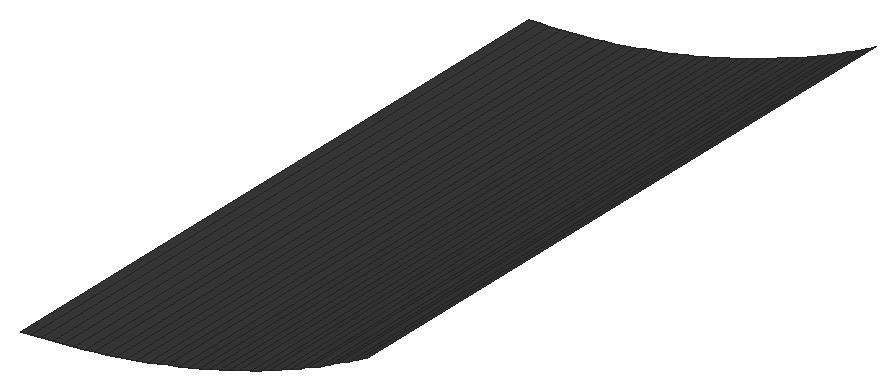
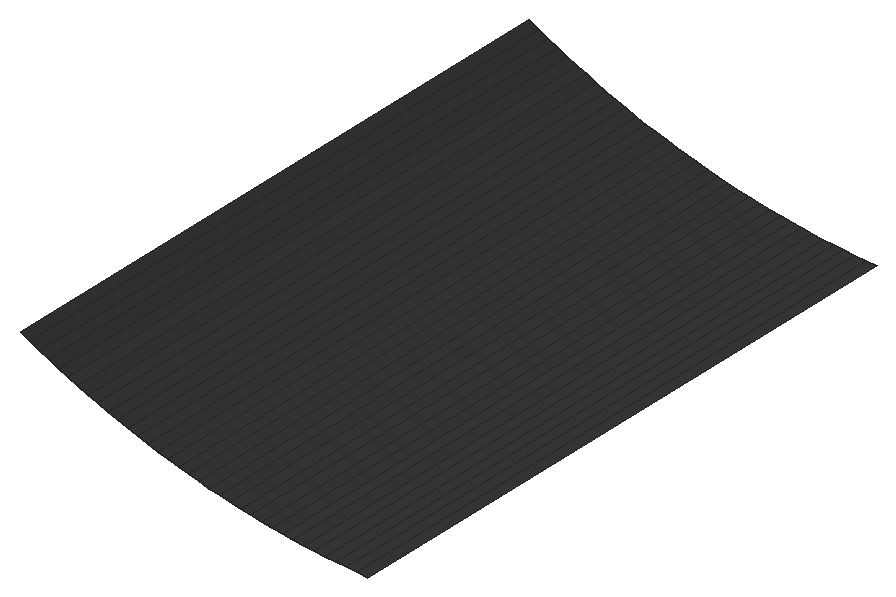
# SketchUp Ruby script. Lengths in inches.
U = 1.inch
M = Sketchup.active_model
def pt(a) = Geom::Point3d.new(a.map { |v| v * U })
def face(e, loops, mat)
  f = e.add_face(loops[0].map { |a| pt(a) })
  loops[1..].each { |l| e.add_face(l.map { |a| pt(a) }).erase! }
  f.material = f.back_material = mat if mat
  f
end
# faces: each face lists its corners as indices into pts; further lists are holes
def faces(e, pts, list, mat = nil) = list.each { |f| face(e, (f[0].is_a?(Array) ? f : [f]).map { |l| l.map { |i| pts[i] } }, mat) }
# xy, xz, yz: faces in a plane at the given z, y or x. An outline is a flat list of corners, or four numbers for a rectangle; further outlines are holes
def ring(l) = l.size == 4 ? [[l[0], l[1]], [l[2], l[1]], [l[2], l[3]], [l[0], l[3]]] : l.each_slice(2).to_a
def flat(e, list, mat, &to3) = list.each { |f| face(e, (f[0].is_a?(Array) ? f : [f]).map { |l| ring(l).map { |u, v| to3.(u, v) } }, mat) }
def xy(e, z, list, mat = nil) = flat(e, list, mat) { |x, y| [x, y, z] }
def xz(e, y, list, mat = nil) = flat(e, list, mat) { |x, z| [x, y, z] }
def yz(e, x, list, mat = nil) = flat(e, list, mat) { |y, z| [x, y, z] }
def lines(e, pts, list) = list.each { |a, b| e.add_line(pt(pts[a]), pt(pts[b])) }
# prism: a flat outline (further loops are holes) pulled along v
def prism(e, loops, v, mat = nil)
  f = face(e, loops, mat); d = Geom::Vector3d.new(v.map { |x| x * U })
  f.pushpull(f.normal.samedirection?(d) ? d.length : -d.length)
end
def box(e, o, s, mat = nil) = prism(e, [[o, [o[0] + s[0], o[1], o[2]], [o[0] + s[0], o[1] + s[1], o[2]], [o[0], o[1] + s[1], o[2]]]], [0, 0, s[2]], mat)
def at(x, y, z, deg = 0) = Geom::Transformation.translation(pt([x, y, z])) * Geom::Transformation.rotation(ORIGIN, Z_AXIS, deg.degrees)
def axes(o, x, y, z) = Geom::Transformation.new([*x, 0, *y, 0, *z, 0, *pt(o).to_a, 1])
def part(name) = M.definitions.add(name)
# library, detail: a bought-in or finely detailed component or shape, given as its bounding box
def library(name, o, s) = part(name).tap { |d| box(d.entities, o, s) }
def detail(e, o, s) = box(e.add_group.entities, o, s)
def put(e, d, t, mat = nil) = e.add_instance(d, t).tap { |i| i.material = mat if mat }
def group(e, t, mat = nil) = e.add_group.tap { |g| g.transformation = t; g.material = mat if mat }.entities
root = M.entities
M.materials.add("1496 AP 8293 CARBON COPY").color = [58, 58, 58]
p = [[291.94,71,143.02],[292.18,71,143.04],[292.18,85,143.04],[291.94,85,143.02],[292.41,71,143.06],[292.41,85,143.06],
  [292.65,71,143.08],[292.65,85,143.08],[292.88,71,143.1],[292.88,85,143.1],[293.12,71,143.125],[293.12,85,143.125],
  [293.35,71,143.15],[293.35,85,143.15],[293.58,71,143.1875],[293.58,85,143.1875],[293.82,71,143.22],[293.82,85,143.22],
  [294.05,71,143.26],[294.05,85,143.26],[294.28,71,143.3],[294.28,85,143.3],[294.51,71,143.35],[294.51,85,143.35],
  [294.74,71,143.39],[294.74,85,143.39],[294.97,71,143.44],[294.97,85,143.44],[295.2,71,143.5],[295.2,85,143.5],
  [295.43,71,143.55],[295.43,85,143.55],[295.66,71,143.61],[295.66,85,143.61],[295.89,71,143.68],[295.89,85,143.68],
  [296.11,71,143.74],[296.11,85,143.74],[296.34,71,143.81],[296.34,85,143.81],[296.5625,71,143.88],[296.5625,85,143.88],
  [296.79,71,143.96],[296.79,85,143.96],[297.01,71,144.03],[297.01,85,144.03],[297.23,71,144.11],[297.23,85,144.11],
  [297.45,71,144.2],[297.45,85,144.2],[297.67,71,144.28],[297.67,85,144.28],[297.89,71,144.37],[297.89,85,144.37],
  [298.11,71,144.46],[298.11,85,144.46],[298.32,71,144.56],[298.32,85,144.56],[298.54,71,144.65],[298.54,85,144.65],
  [298.75,71,144.75],[298.75,85,144.75],[298.96,71,144.86],[298.96,85,144.86],[299.17,71,144.96],[299.17,85,144.96],
  [299.38,71,145.07],[299.38,85,145.07],[299.59,71,145.18],[299.59,85,145.18]]
faces(root,p,[[0,1,2,3],[1,4,5,2],[4,6,7,5],[6,8,9,7],[8,10,11,9],[10,12,13,11],[12,14,15,13],[14,16,17,15],
  [16,18,19,17],[18,20,21,19],[20,22,23,21],[22,24,25,23],[24,26,27,25],[26,28,29,27],[28,30,31,29],[30,32,33,31],
  [32,34,35,33],[34,36,37,35],[36,38,39,37],[38,40,41,39],[40,42,43,41],[42,44,45,43],[44,46,47,45],[46,48,49,47],
  [48,50,51,49],[50,52,53,51],[52,54,55,53],[54,56,57,55],[56,58,59,57],[58,60,61,59],[60,62,63,61],[62,64,65,63],
  [64,66,67,65],[66,68,69,67]],"1496 AP 8293 CARBON COPY")
